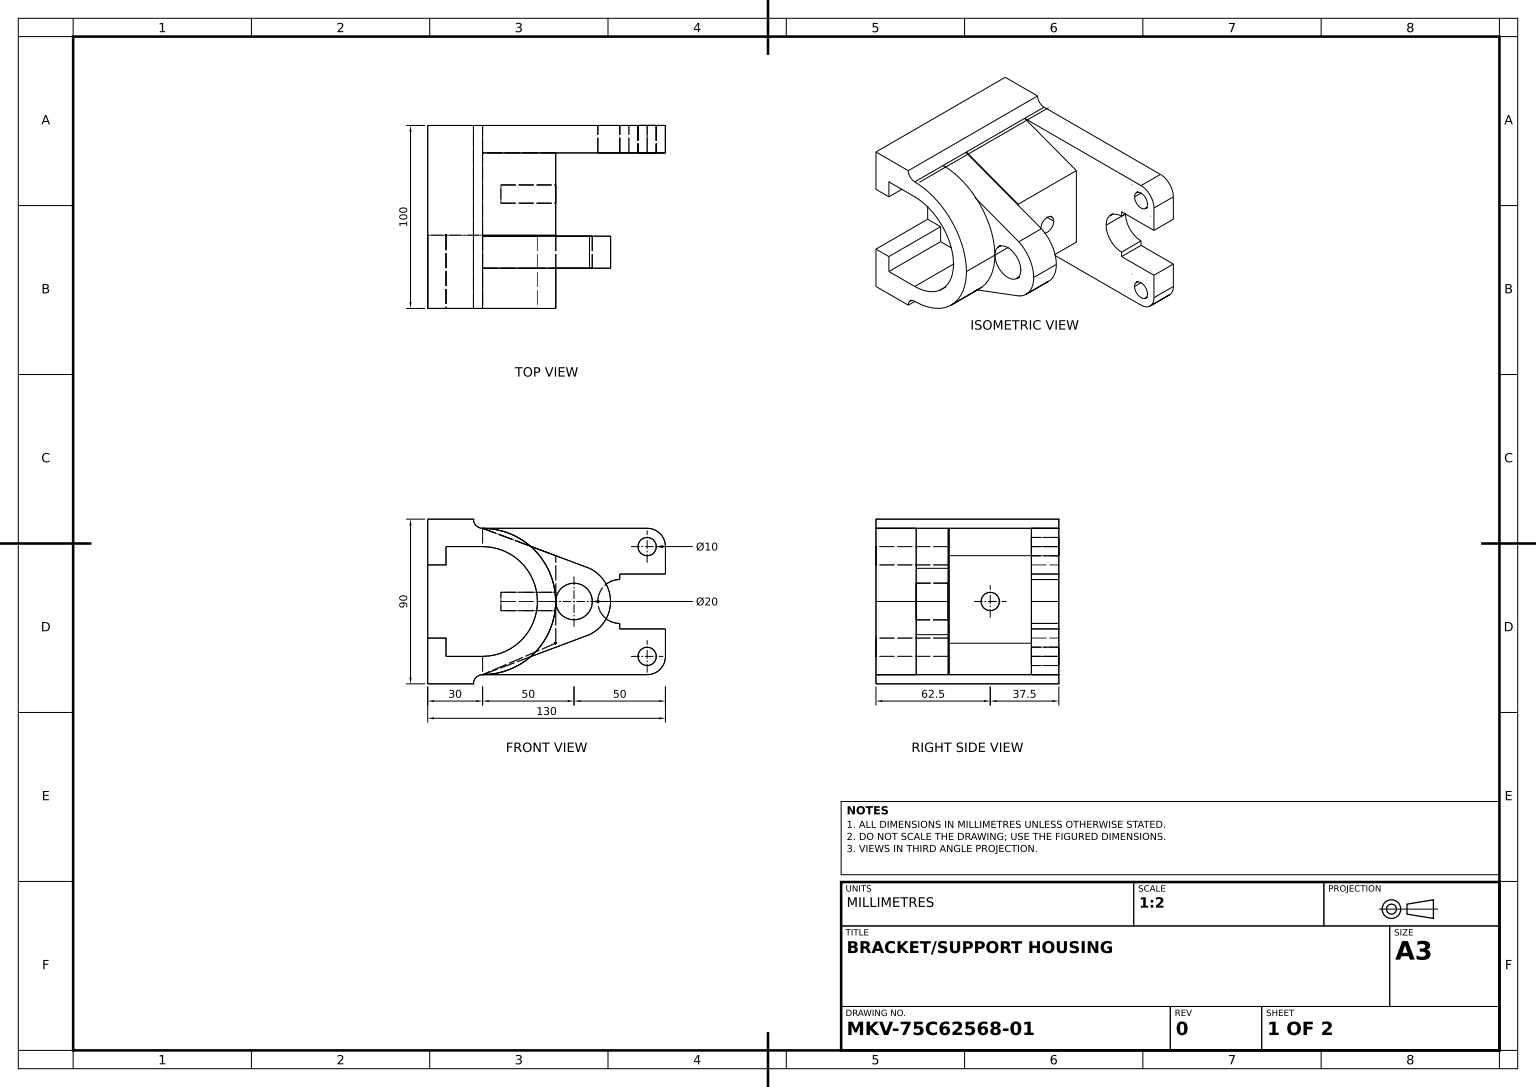
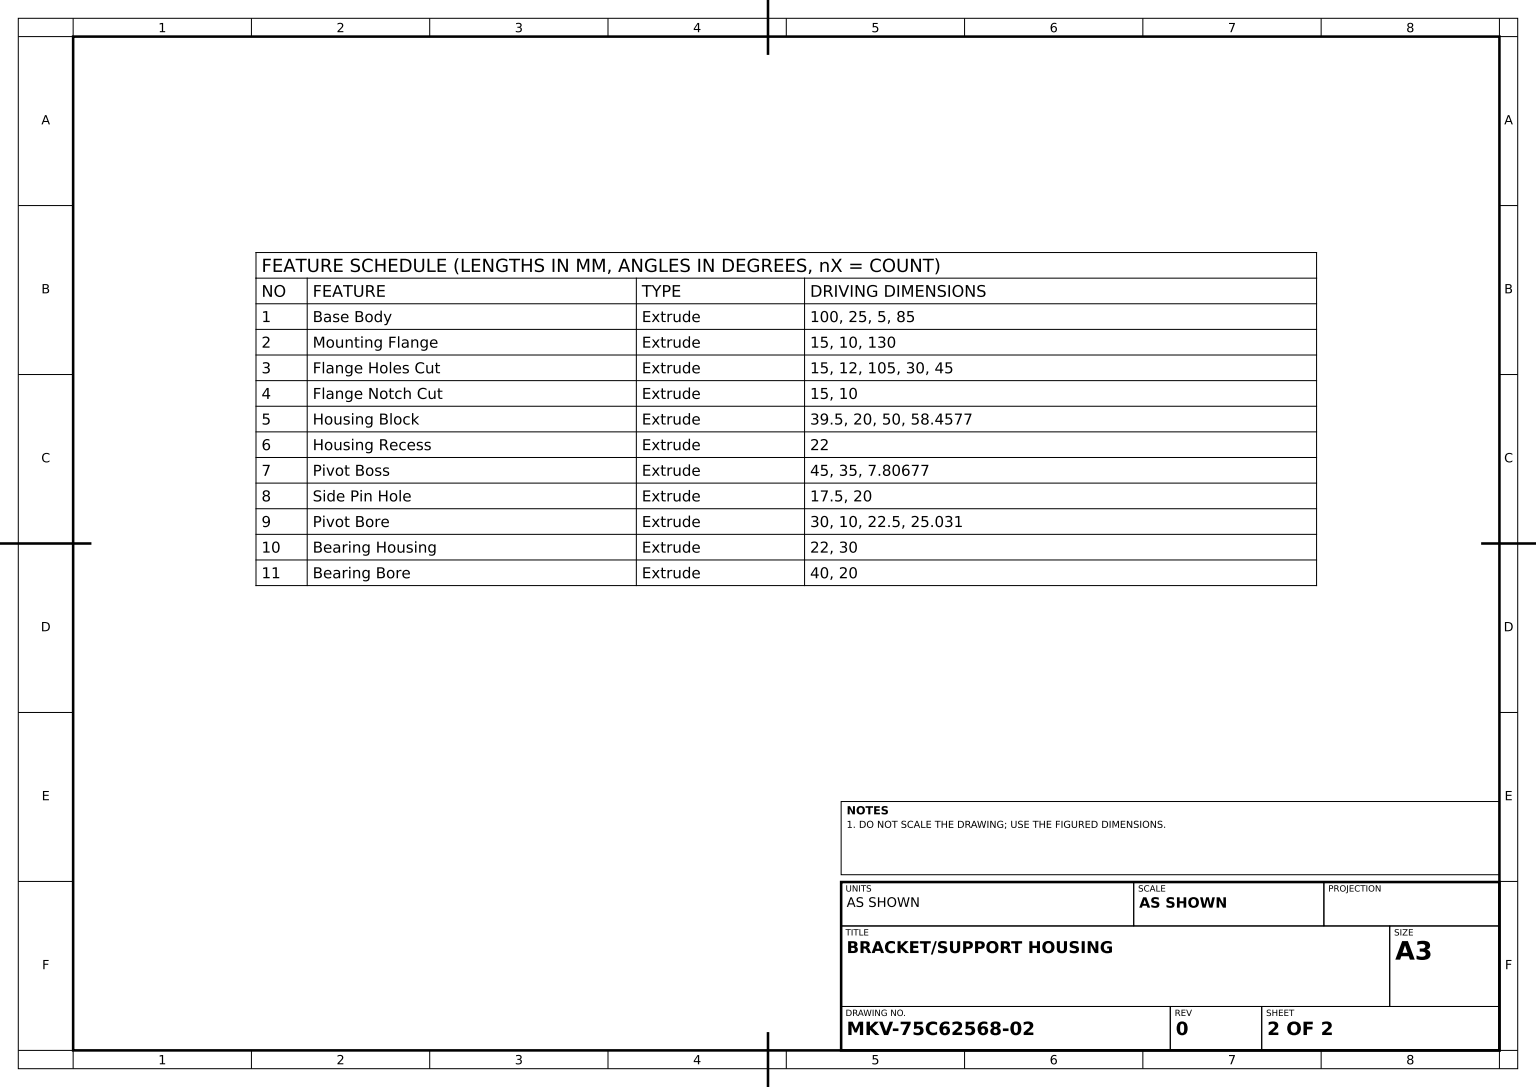
ISO-10303-21;
HEADER;
FILE_DESCRIPTION((''),'2;1');
FILE_NAME('','',(''),(''),'','','');
FILE_SCHEMA(('AUTOMOTIVE_DESIGN'));
ENDSEC;
DATA;
#1=APPLICATION_CONTEXT('');
#2=PRODUCT_CONTEXT('',#1,'mechanical');
#3=PRODUCT('','','',(#2));
#4=PRODUCT_DEFINITION_FORMATION('','',#3);
#5=PRODUCT_DEFINITION_CONTEXT('',#1,'design');
#6=PRODUCT_DEFINITION('','',#4,#5);
#7=PRODUCT_DEFINITION_SHAPE('','',#6);
#8=(LENGTH_UNIT()NAMED_UNIT(*)SI_UNIT(.MILLI.,.METRE.));
#9=(NAMED_UNIT(*)PLANE_ANGLE_UNIT()SI_UNIT($,.RADIAN.));
#10=(NAMED_UNIT(*)SI_UNIT($,.STERADIAN.)SOLID_ANGLE_UNIT());
#11=UNCERTAINTY_MEASURE_WITH_UNIT(LENGTH_MEASURE(1.E-05),#8,'distance_accuracy_value','');
#12=(GEOMETRIC_REPRESENTATION_CONTEXT(3)GLOBAL_UNCERTAINTY_ASSIGNED_CONTEXT((#11))GLOBAL_UNIT_ASSIGNED_CONTEXT((#8,#9,#10))REPRESENTATION_CONTEXT('',''));
#13=CARTESIAN_POINT('',(10.,15.,100.));
#14=VERTEX_POINT('',#13);
#15=CARTESIAN_POINT('',(30.,15.,100.));
#16=VERTEX_POINT('',#15);
#17=DIRECTION('',(1.,0.,0.));
#18=VECTOR('',#17,1000.);
#19=LINE('',#15,#18);
#20=EDGE_CURVE('',#14,#16,#19,.T.);
#21=ORIENTED_EDGE('',*,*,#20,.T.);
#22=CARTESIAN_POINT('',(30.,15.,60.5));
#23=VERTEX_POINT('',#22);
#24=CARTESIAN_POINT('',(30.,15.,78.));
#25=DIRECTION('',(0.,0.,1.));
#26=VECTOR('',#25,1000.);
#27=LINE('',#24,#26);
#28=EDGE_CURVE('',#23,#16,#27,.T.);
#29=ORIENTED_EDGE('',*,*,#28,.F.);
#30=CARTESIAN_POINT('',(30.,15.,60.));
#31=VERTEX_POINT('',#30);
#32=LINE('',#30,#26);
#33=EDGE_CURVE('',#31,#23,#32,.T.);
#34=ORIENTED_EDGE('',*,*,#33,.F.);
#35=CARTESIAN_POINT('',(10.,15.,60.));
#36=VERTEX_POINT('',#35);
#37=LINE('',#30,#18);
#38=EDGE_CURVE('',#36,#31,#37,.T.);
#39=ORIENTED_EDGE('',*,*,#38,.F.);
#40=LINE('',#35,#26);
#41=EDGE_CURVE('',#36,#14,#40,.T.);
#42=ORIENTED_EDGE('',*,*,#41,.T.);
#43=EDGE_LOOP('',(#21,#29,#34,#39,#42));
#44=FACE_OUTER_BOUND('',#43,.T.);
#45=DIRECTION('',(0.,-1.,0.));
#46=DIRECTION('',(0.,0.,-1.));
#47=AXIS2_PLACEMENT_3D('',#30,#45,#46);
#48=PLANE('',#47);
#49=ADVANCED_FACE('',(#44),#48,.F.);
#50=CARTESIAN_POINT('',(70.,45.,78.));
#51=VERTEX_POINT('',#50);
#52=CARTESIAN_POINT('',(70.,45.,100.));
#53=VERTEX_POINT('',#52);
#54=LINE('',#50,#26);
#55=EDGE_CURVE('',#51,#53,#54,.T.);
#56=ORIENTED_EDGE('',*,*,#55,.F.);
#57=CARTESIAN_POINT('',(56.260379,75.172711,78.));
#58=VERTEX_POINT('',#57);
#59=CARTESIAN_POINT('',(30.,45.,78.));
#60=AXIS2_PLACEMENT_3D('',#59,#25,#17);
#61=CIRCLE('',#60,40.);
#62=EDGE_CURVE('',#51,#58,#61,.T.);
#63=ORIENTED_EDGE('',*,*,#62,.T.);
#64=CARTESIAN_POINT('',(30.,85.,78.));
#65=VERTEX_POINT('',#64);
#66=EDGE_CURVE('',#58,#65,#61,.T.);
#67=ORIENTED_EDGE('',*,*,#66,.T.);
#68=CARTESIAN_POINT('',(30.,85.,100.));
#69=VERTEX_POINT('',#68);
#70=VECTOR('',#46,1000.);
#71=LINE('',#68,#70);
#72=EDGE_CURVE('',#69,#65,#71,.T.);
#73=ORIENTED_EDGE('',*,*,#72,.F.);
#74=CARTESIAN_POINT('',(30.,45.,100.));
#75=AXIS2_PLACEMENT_3D('',#74,#25,#17);
#76=CIRCLE('',#75,40.);
#77=EDGE_CURVE('',#53,#69,#76,.T.);
#78=ORIENTED_EDGE('',*,*,#77,.F.);
#79=EDGE_LOOP('',(#56,#63,#67,#73,#78));
#80=FACE_OUTER_BOUND('',#79,.T.);
#81=CYLINDRICAL_SURFACE('',#60,40.);
#82=ADVANCED_FACE('',(#80),#81,.T.);
#83=CARTESIAN_POINT('',(0.,90.,100.));
#84=VERTEX_POINT('',#83);
#85=CARTESIAN_POINT('',(0.,90.,0.));
#86=VERTEX_POINT('',#85);
#87=LINE('',#83,#70);
#88=EDGE_CURVE('',#84,#86,#87,.T.);
#89=ORIENTED_EDGE('',*,*,#88,.F.);
#90=CARTESIAN_POINT('',(25.,90.,100.));
#91=VERTEX_POINT('',#90);
#92=DIRECTION('',(-1.,0.,0.));
#93=VECTOR('',#92,1000.);
#94=LINE('',#83,#93);
#95=EDGE_CURVE('',#91,#84,#94,.T.);
#96=ORIENTED_EDGE('',*,*,#95,.F.);
#97=CARTESIAN_POINT('',(25.,90.,0.));
#98=VERTEX_POINT('',#97);
#99=LINE('',#90,#70);
#100=EDGE_CURVE('',#91,#98,#99,.T.);
#101=ORIENTED_EDGE('',*,*,#100,.T.);
#102=LINE('',#85,#93);
#103=EDGE_CURVE('',#98,#86,#102,.T.);
#104=ORIENTED_EDGE('',*,*,#103,.T.);
#105=EDGE_LOOP('',(#89,#96,#101,#104));
#106=FACE_OUTER_BOUND('',#105,.T.);
#107=AXIS2_PLACEMENT_3D('',#83,#45,#46);
#108=PLANE('',#107);
#109=ADVANCED_FACE('',(#106),#108,.F.);
#110=CARTESIAN_POINT('',(93.,45.,0.));
#111=VERTEX_POINT('',#110);
#112=CARTESIAN_POINT('',(105.,57.,0.));
#113=VERTEX_POINT('',#112);
#114=CARTESIAN_POINT('',(105.,45.,0.));
#115=AXIS2_PLACEMENT_3D('',#114,#46,#92);
#116=CIRCLE('',#115,12.);
#117=EDGE_CURVE('',#111,#113,#116,.T.);
#118=ORIENTED_EDGE('',*,*,#117,.T.);
#119=CARTESIAN_POINT('',(105.,57.,15.));
#120=VERTEX_POINT('',#119);
#121=LINE('',#119,#70);
#122=EDGE_CURVE('',#120,#113,#121,.T.);
#123=ORIENTED_EDGE('',*,*,#122,.F.);
#124=CARTESIAN_POINT('',(93.,45.,15.));
#125=VERTEX_POINT('',#124);
#126=CARTESIAN_POINT('',(105.,45.,15.));
#127=AXIS2_PLACEMENT_3D('',#126,#46,#92);
#128=CIRCLE('',#127,12.);
#129=EDGE_CURVE('',#125,#120,#128,.T.);
#130=ORIENTED_EDGE('',*,*,#129,.F.);
#131=LINE('',#124,#70);
#132=EDGE_CURVE('',#125,#111,#131,.T.);
#133=ORIENTED_EDGE('',*,*,#132,.T.);
#134=EDGE_LOOP('',(#118,#123,#130,#133));
#135=FACE_OUTER_BOUND('',#134,.T.);
#136=CYLINDRICAL_SURFACE('',#127,12.);
#137=ADVANCED_FACE('',(#135),#136,.F.);
#138=CARTESIAN_POINT('',(30.,85.,0.));
#139=VERTEX_POINT('',#138);
#140=CARTESIAN_POINT('',(120.,85.,0.));
#141=VERTEX_POINT('',#140);
#142=LINE('',#140,#18);
#143=EDGE_CURVE('',#139,#141,#142,.T.);
#144=ORIENTED_EDGE('',*,*,#143,.F.);
#145=CARTESIAN_POINT('',(30.,85.,15.));
#146=VERTEX_POINT('',#145);
#147=LINE('',#145,#70);
#148=EDGE_CURVE('',#146,#139,#147,.T.);
#149=ORIENTED_EDGE('',*,*,#148,.F.);
#150=CARTESIAN_POINT('',(120.,85.,15.));
#151=VERTEX_POINT('',#150);
#152=LINE('',#150,#18);
#153=EDGE_CURVE('',#146,#151,#152,.T.);
#154=ORIENTED_EDGE('',*,*,#153,.T.);
#155=LINE('',#150,#70);
#156=EDGE_CURVE('',#151,#141,#155,.T.);
#157=ORIENTED_EDGE('',*,*,#156,.T.);
#158=EDGE_LOOP('',(#144,#149,#154,#157));
#159=FACE_OUTER_BOUND('',#158,.T.);
#160=DIRECTION('',(0.,1.,0.));
#161=AXIS2_PLACEMENT_3D('',#150,#160,#25);
#162=PLANE('',#161);
#163=ADVANCED_FACE('',(#159),#162,.T.);
#164=CARTESIAN_POINT('',(0.,65.,100.));
#165=VERTEX_POINT('',#164);
#166=CARTESIAN_POINT('',(0.,0.,100.));
#167=VECTOR('',#45,1000.);
#168=LINE('',#166,#167);
#169=EDGE_CURVE('',#84,#165,#168,.T.);
#170=ORIENTED_EDGE('',*,*,#169,.F.);
#171=ORIENTED_EDGE('',*,*,#88,.T.);
#172=CARTESIAN_POINT('',(0.,0.,0.));
#173=VERTEX_POINT('',#172);
#174=LINE('',#172,#167);
#175=EDGE_CURVE('',#86,#173,#174,.T.);
#176=ORIENTED_EDGE('',*,*,#175,.T.);
#177=VERTEX_POINT('',#166);
#178=LINE('',#166,#70);
#179=EDGE_CURVE('',#177,#173,#178,.T.);
#180=ORIENTED_EDGE('',*,*,#179,.F.);
#181=CARTESIAN_POINT('',(0.,25.,100.));
#182=VERTEX_POINT('',#181);
#183=EDGE_CURVE('',#182,#177,#168,.T.);
#184=ORIENTED_EDGE('',*,*,#183,.F.);
#185=CARTESIAN_POINT('',(0.,25.,60.));
#186=VERTEX_POINT('',#185);
#187=LINE('',#185,#26);
#188=EDGE_CURVE('',#186,#182,#187,.T.);
#189=ORIENTED_EDGE('',*,*,#188,.F.);
#190=CARTESIAN_POINT('',(0.,65.,60.));
#191=VERTEX_POINT('',#190);
#192=LINE('',#185,#167);
#193=EDGE_CURVE('',#191,#186,#192,.T.);
#194=ORIENTED_EDGE('',*,*,#193,.F.);
#195=LINE('',#190,#26);
#196=EDGE_CURVE('',#191,#165,#195,.T.);
#197=ORIENTED_EDGE('',*,*,#196,.T.);
#198=EDGE_LOOP('',(#170,#171,#176,#180,#184,#189,#194,#197));
#199=FACE_OUTER_BOUND('',#198,.T.);
#200=AXIS2_PLACEMENT_3D('',#166,#17,#46);
#201=PLANE('',#200);
#202=ADVANCED_FACE('',(#199),#201,.F.);
#203=CARTESIAN_POINT('',(70.,22.193233,15.));
#204=VERTEX_POINT('',#203);
#205=CARTESIAN_POINT('',(30.,5.,15.));
#206=VERTEX_POINT('',#205);
#207=CARTESIAN_POINT('',(2.864291,-6.663764,15.));
#208=DIRECTION('',(-0.918725582,-0.394896576,0.));
#209=VECTOR('',#208,1000.);
#210=LINE('',#207,#209);
#211=EDGE_CURVE('',#204,#206,#210,.T.);
#212=ORIENTED_EDGE('',*,*,#211,.F.);
#213=CARTESIAN_POINT('',(70.,22.193233,60.));
#214=VERTEX_POINT('',#213);
#215=LINE('',#213,#70);
#216=EDGE_CURVE('',#214,#204,#215,.T.);
#217=ORIENTED_EDGE('',*,*,#216,.F.);
#218=CARTESIAN_POINT('',(30.,5.,60.));
#219=VERTEX_POINT('',#218);
#220=CARTESIAN_POINT('',(2.864291,-6.663764,60.));
#221=LINE('',#220,#209);
#222=EDGE_CURVE('',#214,#219,#221,.T.);
#223=ORIENTED_EDGE('',*,*,#222,.T.);
#224=LINE('',#218,#70);
#225=EDGE_CURVE('',#219,#206,#224,.T.);
#226=ORIENTED_EDGE('',*,*,#225,.T.);
#227=EDGE_LOOP('',(#212,#217,#223,#226));
#228=FACE_OUTER_BOUND('',#227,.T.);
#229=DIRECTION('',(0.394896576,-0.918725582,0.));
#230=DIRECTION('',(0.918725582,0.394896576,0.));
#231=AXIS2_PLACEMENT_3D('',#220,#229,#230);
#232=PLANE('',#231);
#233=ADVANCED_FACE('',(#228),#232,.T.);
#234=CARTESIAN_POINT('',(105.,60.,0.));
#235=VERTEX_POINT('',#234);
#236=CARTESIAN_POINT('',(130.,60.,0.));
#237=VERTEX_POINT('',#236);
#238=LINE('',#234,#18);
#239=EDGE_CURVE('',#235,#237,#238,.T.);
#240=ORIENTED_EDGE('',*,*,#239,.T.);
#241=CARTESIAN_POINT('',(130.,60.,15.));
#242=VERTEX_POINT('',#241);
#243=LINE('',#241,#70);
#244=EDGE_CURVE('',#242,#237,#243,.T.);
#245=ORIENTED_EDGE('',*,*,#244,.F.);
#246=CARTESIAN_POINT('',(105.,60.,15.));
#247=VERTEX_POINT('',#246);
#248=LINE('',#246,#18);
#249=EDGE_CURVE('',#247,#242,#248,.T.);
#250=ORIENTED_EDGE('',*,*,#249,.F.);
#251=LINE('',#246,#70);
#252=EDGE_CURVE('',#247,#235,#251,.T.);
#253=ORIENTED_EDGE('',*,*,#252,.T.);
#254=EDGE_LOOP('',(#240,#245,#250,#253));
#255=FACE_OUTER_BOUND('',#254,.T.);
#256=AXIS2_PLACEMENT_3D('',#246,#160,#25);
#257=PLANE('',#256);
#258=ADVANCED_FACE('',(#255),#257,.F.);
#259=CARTESIAN_POINT('',(25.,0.,100.));
#260=VERTEX_POINT('',#259);
#261=CARTESIAN_POINT('',(25.,0.,0.));
#262=VERTEX_POINT('',#261);
#263=LINE('',#259,#70);
#264=EDGE_CURVE('',#260,#262,#263,.T.);
#265=ORIENTED_EDGE('',*,*,#264,.F.);
#266=LINE('',#259,#18);
#267=EDGE_CURVE('',#177,#260,#266,.T.);
#268=ORIENTED_EDGE('',*,*,#267,.F.);
#269=ORIENTED_EDGE('',*,*,#179,.T.);
#270=LINE('',#261,#18);
#271=EDGE_CURVE('',#173,#262,#270,.T.);
#272=ORIENTED_EDGE('',*,*,#271,.T.);
#273=EDGE_LOOP('',(#265,#268,#269,#272));
#274=FACE_OUTER_BOUND('',#273,.T.);
#275=AXIS2_PLACEMENT_3D('',#259,#160,#25);
#276=PLANE('',#275);
#277=ADVANCED_FACE('',(#274),#276,.F.);
#278=CARTESIAN_POINT('',(10.,65.,60.));
#279=VERTEX_POINT('',#278);
#280=LINE('',#278,#93);
#281=EDGE_CURVE('',#279,#191,#280,.T.);
#282=ORIENTED_EDGE('',*,*,#281,.F.);
#283=CARTESIAN_POINT('',(10.,65.,100.));
#284=VERTEX_POINT('',#283);
#285=LINE('',#278,#26);
#286=EDGE_CURVE('',#279,#284,#285,.T.);
#287=ORIENTED_EDGE('',*,*,#286,.T.);
#288=LINE('',#283,#93);
#289=EDGE_CURVE('',#284,#165,#288,.T.);
#290=ORIENTED_EDGE('',*,*,#289,.T.);
#291=ORIENTED_EDGE('',*,*,#196,.F.);
#292=EDGE_LOOP('',(#282,#287,#290,#291));
#293=FACE_OUTER_BOUND('',#292,.T.);
#294=AXIS2_PLACEMENT_3D('',#278,#160,#25);
#295=PLANE('',#294);
#296=ADVANCED_FACE('',(#293),#295,.F.);
#297=CARTESIAN_POINT('',(125.,15.,0.));
#298=VERTEX_POINT('',#297);
#299=CARTESIAN_POINT('',(115.,15.,0.));
#300=VERTEX_POINT('',#299);
#301=CARTESIAN_POINT('',(120.,15.,0.));
#302=AXIS2_PLACEMENT_3D('',#301,#25,#17);
#303=CIRCLE('',#302,5.);
#304=EDGE_CURVE('',#298,#300,#303,.T.);
#305=ORIENTED_EDGE('',*,*,#304,.T.);
#306=EDGE_CURVE('',#300,#298,#303,.T.);
#307=ORIENTED_EDGE('',*,*,#306,.T.);
#308=EDGE_LOOP('',(#305,#307));
#309=FACE_BOUND('',#308,.T.);
#310=CARTESIAN_POINT('',(125.,75.,0.));
#311=VERTEX_POINT('',#310);
#312=CARTESIAN_POINT('',(115.,75.,0.));
#313=VERTEX_POINT('',#312);
#314=CARTESIAN_POINT('',(120.,75.,0.));
#315=AXIS2_PLACEMENT_3D('',#314,#25,#17);
#316=CIRCLE('',#315,5.);
#317=EDGE_CURVE('',#311,#313,#316,.T.);
#318=ORIENTED_EDGE('',*,*,#317,.T.);
#319=EDGE_CURVE('',#313,#311,#316,.T.);
#320=ORIENTED_EDGE('',*,*,#319,.T.);
#321=EDGE_LOOP('',(#318,#320));
#322=FACE_BOUND('',#321,.T.);
#323=CARTESIAN_POINT('',(130.,30.,0.));
#324=VERTEX_POINT('',#323);
#325=CARTESIAN_POINT('',(130.,15.,0.));
#326=VERTEX_POINT('',#325);
#327=CARTESIAN_POINT('',(130.,45.,0.));
#328=LINE('',#327,#167);
#329=EDGE_CURVE('',#324,#326,#328,.T.);
#330=ORIENTED_EDGE('',*,*,#329,.T.);
#331=CARTESIAN_POINT('',(120.,5.,0.));
#332=VERTEX_POINT('',#331);
#333=AXIS2_PLACEMENT_3D('',#301,#46,#92);
#334=CIRCLE('',#333,10.);
#335=EDGE_CURVE('',#326,#332,#334,.T.);
#336=ORIENTED_EDGE('',*,*,#335,.T.);
#337=CARTESIAN_POINT('',(30.,5.,0.));
#338=VERTEX_POINT('',#337);
#339=LINE('',#337,#93);
#340=EDGE_CURVE('',#332,#338,#339,.T.);
#341=ORIENTED_EDGE('',*,*,#340,.T.);
#342=CARTESIAN_POINT('',(30.,0.,0.));
#343=AXIS2_PLACEMENT_3D('',#342,#46,#17);
#344=CIRCLE('',#343,5.);
#345=EDGE_CURVE('',#262,#338,#344,.T.);
#346=ORIENTED_EDGE('',*,*,#345,.F.);
#347=ORIENTED_EDGE('',*,*,#271,.F.);
#348=ORIENTED_EDGE('',*,*,#175,.F.);
#349=ORIENTED_EDGE('',*,*,#103,.F.);
#350=CARTESIAN_POINT('',(30.,90.,0.));
#351=AXIS2_PLACEMENT_3D('',#350,#46,#17);
#352=CIRCLE('',#351,5.);
#353=EDGE_CURVE('',#139,#98,#352,.T.);
#354=ORIENTED_EDGE('',*,*,#353,.F.);
#355=ORIENTED_EDGE('',*,*,#143,.T.);
#356=CARTESIAN_POINT('',(130.,75.,0.));
#357=VERTEX_POINT('',#356);
#358=AXIS2_PLACEMENT_3D('',#314,#46,#92);
#359=CIRCLE('',#358,10.);
#360=EDGE_CURVE('',#141,#357,#359,.T.);
#361=ORIENTED_EDGE('',*,*,#360,.T.);
#362=EDGE_CURVE('',#357,#237,#328,.T.);
#363=ORIENTED_EDGE('',*,*,#362,.T.);
#364=ORIENTED_EDGE('',*,*,#239,.F.);
#365=VECTOR('',#160,1000.);
#366=LINE('',#234,#365);
#367=EDGE_CURVE('',#113,#235,#366,.T.);
#368=ORIENTED_EDGE('',*,*,#367,.F.);
#369=ORIENTED_EDGE('',*,*,#117,.F.);
#370=CARTESIAN_POINT('',(105.,33.,0.));
#371=VERTEX_POINT('',#370);
#372=EDGE_CURVE('',#371,#111,#116,.T.);
#373=ORIENTED_EDGE('',*,*,#372,.F.);
#374=CARTESIAN_POINT('',(105.,30.,0.));
#375=VERTEX_POINT('',#374);
#376=LINE('',#370,#365);
#377=EDGE_CURVE('',#375,#371,#376,.T.);
#378=ORIENTED_EDGE('',*,*,#377,.F.);
#379=LINE('',#374,#93);
#380=EDGE_CURVE('',#324,#375,#379,.T.);
#381=ORIENTED_EDGE('',*,*,#380,.F.);
#382=EDGE_LOOP('',(#330,#336,#341,#346,#347,#348,#349,#354,#355,#361,#363,#364,#368,#369,#373,#378,#381));
#383=FACE_OUTER_BOUND('',#382,.T.);
#384=AXIS2_PLACEMENT_3D('',#350,#25,#17);
#385=PLANE('',#384);
#386=ADVANCED_FACE('',(#309,#322,#383),#385,.F.);
#387=CARTESIAN_POINT('',(56.260379,14.827289,78.));
#388=VERTEX_POINT('',#387);
#389=CARTESIAN_POINT('',(88.457667,26.876317,78.));
#390=VERTEX_POINT('',#389);
#391=CARTESIAN_POINT('',(30.,5.,78.));
#392=DIRECTION('',(0.936567609,0.350486966,0.));
#393=VECTOR('',#392,1000.);
#394=LINE('',#391,#393);
#395=EDGE_CURVE('',#388,#390,#394,.T.);
#396=ORIENTED_EDGE('',*,*,#395,.F.);
#397=VERTEX_POINT('',#391);
#398=EDGE_CURVE('',#397,#388,#394,.T.);
#399=ORIENTED_EDGE('',*,*,#398,.F.);
#400=CARTESIAN_POINT('',(30.,5.,60.5));
#401=VERTEX_POINT('',#400);
#402=CARTESIAN_POINT('',(30.,5.,100.));
#403=LINE('',#402,#70);
#404=EDGE_CURVE('',#397,#401,#403,.T.);
#405=ORIENTED_EDGE('',*,*,#404,.T.);
#406=CARTESIAN_POINT('',(88.457667,26.876317,60.5));
#407=VERTEX_POINT('',#406);
#408=LINE('',#400,#393);
#409=EDGE_CURVE('',#401,#407,#408,.T.);
#410=ORIENTED_EDGE('',*,*,#409,.T.);
#411=LINE('',#406,#26);
#412=EDGE_CURVE('',#407,#390,#411,.T.);
#413=ORIENTED_EDGE('',*,*,#412,.T.);
#414=EDGE_LOOP('',(#396,#399,#405,#410,#413));
#415=FACE_OUTER_BOUND('',#414,.T.);
#416=DIRECTION('',(0.350486966,-0.936567609,0.));
#417=AXIS2_PLACEMENT_3D('',#400,#416,#392);
#418=PLANE('',#417);
#419=ADVANCED_FACE('',(#415),#418,.T.);
#420=CARTESIAN_POINT('',(125.,15.,15.));
#421=VERTEX_POINT('',#420);
#422=LINE('',#297,#26);
#423=EDGE_CURVE('',#298,#421,#422,.T.);
#424=ORIENTED_EDGE('',*,*,#423,.T.);
#425=CARTESIAN_POINT('',(115.,15.,15.));
#426=VERTEX_POINT('',#425);
#427=CARTESIAN_POINT('',(120.,15.,15.));
#428=AXIS2_PLACEMENT_3D('',#427,#25,#17);
#429=CIRCLE('',#428,5.);
#430=EDGE_CURVE('',#421,#426,#429,.T.);
#431=ORIENTED_EDGE('',*,*,#430,.T.);
#432=LINE('',#299,#26);
#433=EDGE_CURVE('',#300,#426,#432,.T.);
#434=ORIENTED_EDGE('',*,*,#433,.F.);
#435=ORIENTED_EDGE('',*,*,#304,.F.);
#436=EDGE_LOOP('',(#424,#431,#434,#435));
#437=FACE_OUTER_BOUND('',#436,.T.);
#438=CYLINDRICAL_SURFACE('',#302,5.);
#439=ADVANCED_FACE('',(#437),#438,.F.);
#440=CARTESIAN_POINT('',(30.,75.,60.5));
#441=VERTEX_POINT('',#440);
#442=CARTESIAN_POINT('',(30.,75.,100.));
#443=VERTEX_POINT('',#442);
#444=CARTESIAN_POINT('',(30.,75.,78.));
#445=LINE('',#444,#26);
#446=EDGE_CURVE('',#441,#443,#445,.T.);
#447=ORIENTED_EDGE('',*,*,#446,.F.);
#448=CARTESIAN_POINT('',(60.,45.,60.5));
#449=VERTEX_POINT('',#448);
#450=CARTESIAN_POINT('',(30.,45.,60.5));
#451=AXIS2_PLACEMENT_3D('',#450,#25,#17);
#452=CIRCLE('',#451,30.);
#453=EDGE_CURVE('',#449,#441,#452,.T.);
#454=ORIENTED_EDGE('',*,*,#453,.F.);
#455=CARTESIAN_POINT('',(60.,45.,100.));
#456=VERTEX_POINT('',#455);
#457=CARTESIAN_POINT('',(60.,45.,78.));
#458=LINE('',#457,#26);
#459=EDGE_CURVE('',#449,#456,#458,.T.);
#460=ORIENTED_EDGE('',*,*,#459,.T.);
#461=CIRCLE('',#75,30.);
#462=EDGE_CURVE('',#456,#443,#461,.T.);
#463=ORIENTED_EDGE('',*,*,#462,.T.);
#464=EDGE_LOOP('',(#447,#454,#460,#463));
#465=FACE_OUTER_BOUND('',#464,.T.);
#466=CYLINDRICAL_SURFACE('',#60,30.);
#467=ADVANCED_FACE('',(#465),#466,.F.);
#468=CARTESIAN_POINT('',(105.,30.,15.));
#469=VERTEX_POINT('',#468);
#470=LINE('',#468,#70);
#471=EDGE_CURVE('',#469,#375,#470,.T.);
#472=ORIENTED_EDGE('',*,*,#471,.T.);
#473=ORIENTED_EDGE('',*,*,#377,.T.);
#474=CARTESIAN_POINT('',(105.,33.,15.));
#475=VERTEX_POINT('',#474);
#476=LINE('',#474,#70);
#477=EDGE_CURVE('',#475,#371,#476,.T.);
#478=ORIENTED_EDGE('',*,*,#477,.F.);
#479=LINE('',#474,#365);
#480=EDGE_CURVE('',#469,#475,#479,.T.);
#481=ORIENTED_EDGE('',*,*,#480,.F.);
#482=EDGE_LOOP('',(#472,#473,#478,#481));
#483=FACE_OUTER_BOUND('',#482,.T.);
#484=AXIS2_PLACEMENT_3D('',#474,#92,#25);
#485=PLANE('',#484);
#486=ADVANCED_FACE('',(#483),#485,.F.);
#487=ORIENTED_EDGE('',*,*,#433,.T.);
#488=EDGE_CURVE('',#426,#421,#429,.T.);
#489=ORIENTED_EDGE('',*,*,#488,.T.);
#490=ORIENTED_EDGE('',*,*,#423,.F.);
#491=ORIENTED_EDGE('',*,*,#306,.F.);
#492=EDGE_LOOP('',(#487,#489,#490,#491));
#493=FACE_OUTER_BOUND('',#492,.T.);
#494=ADVANCED_FACE('',(#493),#438,.F.);
#495=ORIENTED_EDGE('',*,*,#395,.T.);
#496=CARTESIAN_POINT('',(100.,45.,78.));
#497=VERTEX_POINT('',#496);
#498=CARTESIAN_POINT('',(80.,45.,78.));
#499=AXIS2_PLACEMENT_3D('',#498,#25,#17);
#500=CIRCLE('',#499,20.);
#501=EDGE_CURVE('',#390,#497,#500,.T.);
#502=ORIENTED_EDGE('',*,*,#501,.T.);
#503=CARTESIAN_POINT('',(88.457667,63.123683,78.));
#504=VERTEX_POINT('',#503);
#505=EDGE_CURVE('',#497,#504,#500,.T.);
#506=ORIENTED_EDGE('',*,*,#505,.T.);
#507=DIRECTION('',(-0.936567609,0.350486966,0.));
#508=VECTOR('',#507,1000.);
#509=LINE('',#503,#508);
#510=EDGE_CURVE('',#504,#58,#509,.T.);
#511=ORIENTED_EDGE('',*,*,#510,.T.);
#512=ORIENTED_EDGE('',*,*,#62,.F.);
#513=CARTESIAN_POINT('',(90.,45.,78.));
#514=VERTEX_POINT('',#513);
#515=CIRCLE('',#499,10.);
#516=EDGE_CURVE('',#514,#51,#515,.T.);
#517=ORIENTED_EDGE('',*,*,#516,.F.);
#518=EDGE_CURVE('',#51,#514,#515,.T.);
#519=ORIENTED_EDGE('',*,*,#518,.F.);
#520=EDGE_CURVE('',#388,#51,#61,.T.);
#521=ORIENTED_EDGE('',*,*,#520,.F.);
#522=EDGE_LOOP('',(#495,#502,#506,#511,#512,#517,#519,#521));
#523=FACE_OUTER_BOUND('',#522,.T.);
#524=PLANE('',#499);
#525=ADVANCED_FACE('',(#523),#524,.T.);
#526=CARTESIAN_POINT('',(125.,75.,15.));
#527=VERTEX_POINT('',#526);
#528=CARTESIAN_POINT('',(115.,75.,15.));
#529=VERTEX_POINT('',#528);
#530=CARTESIAN_POINT('',(120.,75.,15.));
#531=AXIS2_PLACEMENT_3D('',#530,#25,#17);
#532=CIRCLE('',#531,5.);
#533=EDGE_CURVE('',#527,#529,#532,.T.);
#534=ORIENTED_EDGE('',*,*,#533,.T.);
#535=LINE('',#312,#26);
#536=EDGE_CURVE('',#313,#529,#535,.T.);
#537=ORIENTED_EDGE('',*,*,#536,.F.);
#538=ORIENTED_EDGE('',*,*,#317,.F.);
#539=LINE('',#310,#26);
#540=EDGE_CURVE('',#311,#527,#539,.T.);
#541=ORIENTED_EDGE('',*,*,#540,.T.);
#542=EDGE_LOOP('',(#534,#537,#538,#541));
#543=FACE_OUTER_BOUND('',#542,.T.);
#544=CYLINDRICAL_SURFACE('',#315,5.);
#545=ADVANCED_FACE('',(#543),#544,.F.);
#546=CARTESIAN_POINT('',(130.,75.,15.));
#547=VERTEX_POINT('',#546);
#548=AXIS2_PLACEMENT_3D('',#530,#46,#92);
#549=CIRCLE('',#548,10.);
#550=EDGE_CURVE('',#151,#547,#549,.T.);
#551=ORIENTED_EDGE('',*,*,#550,.T.);
#552=LINE('',#546,#70);
#553=EDGE_CURVE('',#547,#357,#552,.T.);
#554=ORIENTED_EDGE('',*,*,#553,.T.);
#555=ORIENTED_EDGE('',*,*,#360,.F.);
#556=ORIENTED_EDGE('',*,*,#156,.F.);
#557=EDGE_LOOP('',(#551,#554,#555,#556));
#558=FACE_OUTER_BOUND('',#557,.T.);
#559=CYLINDRICAL_SURFACE('',#548,10.);
#560=ADVANCED_FACE('',(#558),#559,.T.);
#561=CARTESIAN_POINT('',(30.,85.,60.5));
#562=VERTEX_POINT('',#561);
#563=LINE('',#561,#167);
#564=EDGE_CURVE('',#562,#441,#563,.T.);
#565=ORIENTED_EDGE('',*,*,#564,.T.);
#566=CARTESIAN_POINT('',(30.,75.,60.));
#567=VERTEX_POINT('',#566);
#568=LINE('',#566,#26);
#569=EDGE_CURVE('',#567,#441,#568,.T.);
#570=ORIENTED_EDGE('',*,*,#569,.F.);
#571=CARTESIAN_POINT('',(30.,85.,60.));
#572=VERTEX_POINT('',#571);
#573=CARTESIAN_POINT('',(30.,0.,60.));
#574=LINE('',#573,#167);
#575=EDGE_CURVE('',#572,#567,#574,.T.);
#576=ORIENTED_EDGE('',*,*,#575,.F.);
#577=EDGE_CURVE('',#562,#572,#71,.T.);
#578=ORIENTED_EDGE('',*,*,#577,.F.);
#579=EDGE_LOOP('',(#565,#570,#576,#578));
#580=FACE_OUTER_BOUND('',#579,.T.);
#581=AXIS2_PLACEMENT_3D('',#68,#92,#25);
#582=PLANE('',#581);
#583=ADVANCED_FACE('',(#580),#582,.F.);
#584=CARTESIAN_POINT('',(40.,45.,42.5));
#585=VERTEX_POINT('',#584);
#586=CARTESIAN_POINT('',(40.,45.,32.5));
#587=VERTEX_POINT('',#586);
#588=CARTESIAN_POINT('',(40.,45.,37.5));
#589=AXIS2_PLACEMENT_3D('',#588,#17,#46);
#590=CIRCLE('',#589,5.);
#591=EDGE_CURVE('',#585,#587,#590,.T.);
#592=ORIENTED_EDGE('',*,*,#591,.F.);
#593=CARTESIAN_POINT('',(70.,45.,42.5));
#594=VERTEX_POINT('',#593);
#595=LINE('',#584,#18);
#596=EDGE_CURVE('',#585,#594,#595,.T.);
#597=ORIENTED_EDGE('',*,*,#596,.T.);
#598=CARTESIAN_POINT('',(70.,45.,32.5));
#599=VERTEX_POINT('',#598);
#600=CARTESIAN_POINT('',(70.,45.,37.5));
#601=AXIS2_PLACEMENT_3D('',#600,#17,#46);
#602=CIRCLE('',#601,5.);
#603=EDGE_CURVE('',#594,#599,#602,.T.);
#604=ORIENTED_EDGE('',*,*,#603,.T.);
#605=LINE('',#586,#18);
#606=EDGE_CURVE('',#587,#599,#605,.T.);
#607=ORIENTED_EDGE('',*,*,#606,.F.);
#608=EDGE_LOOP('',(#592,#597,#604,#607));
#609=FACE_OUTER_BOUND('',#608,.T.);
#610=CYLINDRICAL_SURFACE('',#589,5.);
#611=ADVANCED_FACE('',(#609),#610,.F.);
#612=CARTESIAN_POINT('',(70.,70.031002,60.));
#613=VERTEX_POINT('',#612);
#614=CARTESIAN_POINT('',(70.,70.031002,15.));
#615=VERTEX_POINT('',#614);
#616=LINE('',#612,#70);
#617=EDGE_CURVE('',#613,#615,#616,.T.);
#618=ORIENTED_EDGE('',*,*,#617,.T.);
#619=CARTESIAN_POINT('',(31.586886,84.406148,15.));
#620=LINE('',#619,#508);
#621=EDGE_CURVE('',#615,#146,#620,.T.);
#622=ORIENTED_EDGE('',*,*,#621,.T.);
#623=LINE('',#571,#70);
#624=EDGE_CURVE('',#572,#146,#623,.T.);
#625=ORIENTED_EDGE('',*,*,#624,.F.);
#626=CARTESIAN_POINT('',(31.586886,84.406148,60.));
#627=LINE('',#626,#508);
#628=EDGE_CURVE('',#613,#572,#627,.T.);
#629=ORIENTED_EDGE('',*,*,#628,.F.);
#630=EDGE_LOOP('',(#618,#622,#625,#629));
#631=FACE_OUTER_BOUND('',#630,.T.);
#632=DIRECTION('',(-0.350486966,-0.936567609,0.));
#633=DIRECTION('',(0.936567609,-0.350486966,0.));
#634=AXIS2_PLACEMENT_3D('',#626,#632,#633);
#635=PLANE('',#634);
#636=ADVANCED_FACE('',(#631),#635,.F.);
#637=ORIENTED_EDGE('',*,*,#329,.F.);
#638=CARTESIAN_POINT('',(130.,30.,15.));
#639=VERTEX_POINT('',#638);
#640=LINE('',#638,#70);
#641=EDGE_CURVE('',#639,#324,#640,.T.);
#642=ORIENTED_EDGE('',*,*,#641,.F.);
#643=CARTESIAN_POINT('',(130.,15.,15.));
#644=VERTEX_POINT('',#643);
#645=CARTESIAN_POINT('',(130.,45.,15.));
#646=LINE('',#645,#167);
#647=EDGE_CURVE('',#639,#644,#646,.T.);
#648=ORIENTED_EDGE('',*,*,#647,.T.);
#649=LINE('',#643,#70);
#650=EDGE_CURVE('',#644,#326,#649,.T.);
#651=ORIENTED_EDGE('',*,*,#650,.T.);
#652=EDGE_LOOP('',(#637,#642,#648,#651));
#653=FACE_OUTER_BOUND('',#652,.T.);
#654=AXIS2_PLACEMENT_3D('',#645,#17,#46);
#655=PLANE('',#654);
#656=ADVANCED_FACE('',(#653),#655,.T.);
#657=ORIENTED_EDGE('',*,*,#606,.T.);
#658=EDGE_CURVE('',#599,#594,#602,.T.);
#659=ORIENTED_EDGE('',*,*,#658,.T.);
#660=ORIENTED_EDGE('',*,*,#596,.F.);
#661=EDGE_CURVE('',#587,#585,#590,.T.);
#662=ORIENTED_EDGE('',*,*,#661,.F.);
#663=EDGE_LOOP('',(#657,#659,#660,#662));
#664=FACE_OUTER_BOUND('',#663,.T.);
#665=ADVANCED_FACE('',(#664),#610,.F.);
#666=ORIENTED_EDGE('',*,*,#122,.T.);
#667=ORIENTED_EDGE('',*,*,#367,.T.);
#668=ORIENTED_EDGE('',*,*,#252,.F.);
#669=LINE('',#246,#365);
#670=EDGE_CURVE('',#120,#247,#669,.T.);
#671=ORIENTED_EDGE('',*,*,#670,.F.);
#672=EDGE_LOOP('',(#666,#667,#668,#671));
#673=FACE_OUTER_BOUND('',#672,.T.);
#674=AXIS2_PLACEMENT_3D('',#246,#92,#25);
#675=PLANE('',#674);
#676=ADVANCED_FACE('',(#673),#675,.F.);
#677=CARTESIAN_POINT('',(10.,75.,60.));
#678=VERTEX_POINT('',#677);
#679=CARTESIAN_POINT('',(10.,75.,100.));
#680=VERTEX_POINT('',#679);
#681=LINE('',#677,#26);
#682=EDGE_CURVE('',#678,#680,#681,.T.);
#683=ORIENTED_EDGE('',*,*,#682,.F.);
#684=LINE('',#566,#93);
#685=EDGE_CURVE('',#567,#678,#684,.T.);
#686=ORIENTED_EDGE('',*,*,#685,.F.);
#687=ORIENTED_EDGE('',*,*,#569,.T.);
#688=ORIENTED_EDGE('',*,*,#446,.T.);
#689=LINE('',#442,#93);
#690=EDGE_CURVE('',#443,#680,#689,.T.);
#691=ORIENTED_EDGE('',*,*,#690,.T.);
#692=EDGE_LOOP('',(#683,#686,#687,#688,#691));
#693=FACE_OUTER_BOUND('',#692,.T.);
#694=AXIS2_PLACEMENT_3D('',#566,#160,#25);
#695=PLANE('',#694);
#696=ADVANCED_FACE('',(#693),#695,.F.);
#697=EDGE_CURVE('',#23,#449,#452,.T.);
#698=ORIENTED_EDGE('',*,*,#697,.T.);
#699=ORIENTED_EDGE('',*,*,#453,.T.);
#700=ORIENTED_EDGE('',*,*,#564,.F.);
#701=CARTESIAN_POINT('',(88.457667,63.123683,60.5));
#702=VERTEX_POINT('',#701);
#703=LINE('',#561,#508);
#704=EDGE_CURVE('',#702,#562,#703,.T.);
#705=ORIENTED_EDGE('',*,*,#704,.F.);
#706=CARTESIAN_POINT('',(100.,45.,60.5));
#707=VERTEX_POINT('',#706);
#708=CARTESIAN_POINT('',(80.,45.,60.5));
#709=AXIS2_PLACEMENT_3D('',#708,#25,#17);
#710=CIRCLE('',#709,20.);
#711=EDGE_CURVE('',#707,#702,#710,.T.);
#712=ORIENTED_EDGE('',*,*,#711,.F.);
#713=EDGE_CURVE('',#407,#707,#710,.T.);
#714=ORIENTED_EDGE('',*,*,#713,.F.);
#715=ORIENTED_EDGE('',*,*,#409,.F.);
#716=EDGE_CURVE('',#23,#401,#563,.T.);
#717=ORIENTED_EDGE('',*,*,#716,.F.);
#718=EDGE_LOOP('',(#698,#699,#700,#705,#712,#714,#715,#717));
#719=FACE_OUTER_BOUND('',#718,.T.);
#720=CARTESIAN_POINT('',(70.,45.,60.5));
#721=VERTEX_POINT('',#720);
#722=CARTESIAN_POINT('',(90.,45.,60.5));
#723=VERTEX_POINT('',#722);
#724=CIRCLE('',#709,10.);
#725=EDGE_CURVE('',#721,#723,#724,.T.);
#726=ORIENTED_EDGE('',*,*,#725,.T.);
#727=EDGE_CURVE('',#723,#721,#724,.T.);
#728=ORIENTED_EDGE('',*,*,#727,.T.);
#729=EDGE_LOOP('',(#726,#728));
#730=FACE_BOUND('',#729,.T.);
#731=PLANE('',#709);
#732=ADVANCED_FACE('',(#719,#730),#731,.F.);
#733=ORIENTED_EDGE('',*,*,#471,.F.);
#734=LINE('',#468,#93);
#735=EDGE_CURVE('',#639,#469,#734,.T.);
#736=ORIENTED_EDGE('',*,*,#735,.F.);
#737=ORIENTED_EDGE('',*,*,#641,.T.);
#738=ORIENTED_EDGE('',*,*,#380,.T.);
#739=EDGE_LOOP('',(#733,#736,#737,#738));
#740=FACE_OUTER_BOUND('',#739,.T.);
#741=AXIS2_PLACEMENT_3D('',#468,#45,#17);
#742=PLANE('',#741);
#743=ADVANCED_FACE('',(#740),#742,.F.);
#744=ORIENTED_EDGE('',*,*,#682,.T.);
#745=LINE('',#679,#167);
#746=EDGE_CURVE('',#680,#284,#745,.T.);
#747=ORIENTED_EDGE('',*,*,#746,.T.);
#748=ORIENTED_EDGE('',*,*,#286,.F.);
#749=LINE('',#677,#167);
#750=EDGE_CURVE('',#678,#279,#749,.T.);
#751=ORIENTED_EDGE('',*,*,#750,.F.);
#752=EDGE_LOOP('',(#744,#747,#748,#751));
#753=FACE_OUTER_BOUND('',#752,.T.);
#754=AXIS2_PLACEMENT_3D('',#677,#92,#25);
#755=PLANE('',#754);
#756=ADVANCED_FACE('',(#753),#755,.F.);
#757=EDGE_CURVE('',#397,#388,#61,.T.);
#758=ORIENTED_EDGE('',*,*,#757,.F.);
#759=ORIENTED_EDGE('',*,*,#398,.T.);
#760=EDGE_LOOP('',(#758,#759));
#761=FACE_OUTER_BOUND('',#760,.T.);
#762=CARTESIAN_POINT('',(0.,0.,78.));
#763=AXIS2_PLACEMENT_3D('',#762,#25,#17);
#764=PLANE('',#763);
#765=ADVANCED_FACE('',(#761),#764,.F.);
#766=ORIENTED_EDGE('',*,*,#727,.F.);
#767=LINE('',#722,#26);
#768=EDGE_CURVE('',#723,#514,#767,.T.);
#769=ORIENTED_EDGE('',*,*,#768,.T.);
#770=ORIENTED_EDGE('',*,*,#516,.T.);
#771=LINE('',#720,#26);
#772=EDGE_CURVE('',#721,#51,#771,.T.);
#773=ORIENTED_EDGE('',*,*,#772,.F.);
#774=EDGE_LOOP('',(#766,#769,#770,#773));
#775=FACE_OUTER_BOUND('',#774,.T.);
#776=CYLINDRICAL_SURFACE('',#709,10.);
#777=ADVANCED_FACE('',(#775),#776,.F.);
#778=ORIENTED_EDGE('',*,*,#591,.T.);
#779=ORIENTED_EDGE('',*,*,#661,.T.);
#780=EDGE_LOOP('',(#778,#779));
#781=FACE_OUTER_BOUND('',#780,.T.);
#782=PLANE('',#589);
#783=ADVANCED_FACE('',(#781),#782,.T.);
#784=ORIENTED_EDGE('',*,*,#41,.F.);
#785=CARTESIAN_POINT('',(10.,25.,60.));
#786=VERTEX_POINT('',#785);
#787=LINE('',#35,#167);
#788=EDGE_CURVE('',#786,#36,#787,.T.);
#789=ORIENTED_EDGE('',*,*,#788,.F.);
#790=CARTESIAN_POINT('',(10.,25.,100.));
#791=VERTEX_POINT('',#790);
#792=LINE('',#785,#26);
#793=EDGE_CURVE('',#786,#791,#792,.T.);
#794=ORIENTED_EDGE('',*,*,#793,.T.);
#795=LINE('',#13,#167);
#796=EDGE_CURVE('',#791,#14,#795,.T.);
#797=ORIENTED_EDGE('',*,*,#796,.T.);
#798=EDGE_LOOP('',(#784,#789,#794,#797));
#799=FACE_OUTER_BOUND('',#798,.T.);
#800=AXIS2_PLACEMENT_3D('',#35,#92,#25);
#801=PLANE('',#800);
#802=ADVANCED_FACE('',(#799),#801,.F.);
#803=ORIENTED_EDGE('',*,*,#768,.F.);
#804=ORIENTED_EDGE('',*,*,#725,.F.);
#805=ORIENTED_EDGE('',*,*,#772,.T.);
#806=ORIENTED_EDGE('',*,*,#518,.T.);
#807=EDGE_LOOP('',(#803,#804,#805,#806));
#808=FACE_OUTER_BOUND('',#807,.T.);
#809=ADVANCED_FACE('',(#808),#776,.F.);
#810=EDGE_CURVE('',#31,#219,#574,.T.);
#811=ORIENTED_EDGE('',*,*,#810,.F.);
#812=ORIENTED_EDGE('',*,*,#33,.T.);
#813=ORIENTED_EDGE('',*,*,#716,.T.);
#814=EDGE_CURVE('',#401,#219,#403,.T.);
#815=ORIENTED_EDGE('',*,*,#814,.T.);
#816=EDGE_LOOP('',(#811,#812,#813,#815));
#817=FACE_OUTER_BOUND('',#816,.T.);
#818=ADVANCED_FACE('',(#817),#582,.F.);
#819=ORIENTED_EDGE('',*,*,#793,.F.);
#820=LINE('',#785,#18);
#821=EDGE_CURVE('',#186,#786,#820,.T.);
#822=ORIENTED_EDGE('',*,*,#821,.F.);
#823=ORIENTED_EDGE('',*,*,#188,.T.);
#824=LINE('',#790,#18);
#825=EDGE_CURVE('',#182,#791,#824,.T.);
#826=ORIENTED_EDGE('',*,*,#825,.T.);
#827=EDGE_LOOP('',(#819,#822,#823,#826));
#828=FACE_OUTER_BOUND('',#827,.T.);
#829=AXIS2_PLACEMENT_3D('',#785,#45,#17);
#830=PLANE('',#829);
#831=ADVANCED_FACE('',(#828),#830,.F.);
#832=ORIENTED_EDGE('',*,*,#66,.F.);
#833=VECTOR('',#633,1000.);
#834=LINE('',#64,#833);
#835=EDGE_CURVE('',#65,#58,#834,.T.);
#836=ORIENTED_EDGE('',*,*,#835,.F.);
#837=EDGE_LOOP('',(#832,#836));
#838=FACE_OUTER_BOUND('',#837,.T.);
#839=ADVANCED_FACE('',(#838),#764,.F.);
#840=ORIENTED_EDGE('',*,*,#510,.F.);
#841=LINE('',#701,#26);
#842=EDGE_CURVE('',#702,#504,#841,.T.);
#843=ORIENTED_EDGE('',*,*,#842,.F.);
#844=ORIENTED_EDGE('',*,*,#704,.T.);
#845=EDGE_CURVE('',#65,#562,#71,.T.);
#846=ORIENTED_EDGE('',*,*,#845,.F.);
#847=ORIENTED_EDGE('',*,*,#835,.T.);
#848=EDGE_LOOP('',(#840,#843,#844,#846,#847));
#849=FACE_OUTER_BOUND('',#848,.T.);
#850=DIRECTION('',(0.350486966,0.936567609,0.));
#851=AXIS2_PLACEMENT_3D('',#561,#850,#507);
#852=PLANE('',#851);
#853=ADVANCED_FACE('',(#849),#852,.T.);
#854=CARTESIAN_POINT('',(70.,0.,60.));
#855=LINE('',#854,#365);
#856=EDGE_CURVE('',#214,#613,#855,.T.);
#857=ORIENTED_EDGE('',*,*,#856,.T.);
#858=ORIENTED_EDGE('',*,*,#628,.T.);
#859=ORIENTED_EDGE('',*,*,#575,.T.);
#860=ORIENTED_EDGE('',*,*,#685,.T.);
#861=ORIENTED_EDGE('',*,*,#750,.T.);
#862=ORIENTED_EDGE('',*,*,#281,.T.);
#863=ORIENTED_EDGE('',*,*,#193,.T.);
#864=ORIENTED_EDGE('',*,*,#821,.T.);
#865=ORIENTED_EDGE('',*,*,#788,.T.);
#866=ORIENTED_EDGE('',*,*,#38,.T.);
#867=ORIENTED_EDGE('',*,*,#810,.T.);
#868=ORIENTED_EDGE('',*,*,#222,.F.);
#869=EDGE_LOOP('',(#857,#858,#859,#860,#861,#862,#863,#864,#865,#866,#867,#868));
#870=FACE_OUTER_BOUND('',#869,.T.);
#871=CARTESIAN_POINT('',(0.,0.,60.));
#872=AXIS2_PLACEMENT_3D('',#871,#25,#17);
#873=PLANE('',#872);
#874=ADVANCED_FACE('',(#870),#873,.T.);
#875=ORIENTED_EDGE('',*,*,#842,.T.);
#876=ORIENTED_EDGE('',*,*,#505,.F.);
#877=LINE('',#706,#26);
#878=EDGE_CURVE('',#707,#497,#877,.T.);
#879=ORIENTED_EDGE('',*,*,#878,.F.);
#880=ORIENTED_EDGE('',*,*,#711,.T.);
#881=EDGE_LOOP('',(#875,#876,#879,#880));
#882=FACE_OUTER_BOUND('',#881,.T.);
#883=CYLINDRICAL_SURFACE('',#709,20.);
#884=ADVANCED_FACE('',(#882),#883,.T.);
#885=ORIENTED_EDGE('',*,*,#267,.T.);
#886=VERTEX_POINT('',#402);
#887=CARTESIAN_POINT('',(30.,0.,100.));
#888=AXIS2_PLACEMENT_3D('',#887,#46,#17);
#889=CIRCLE('',#888,5.);
#890=EDGE_CURVE('',#260,#886,#889,.T.);
#891=ORIENTED_EDGE('',*,*,#890,.T.);
#892=EDGE_CURVE('',#886,#53,#76,.T.);
#893=ORIENTED_EDGE('',*,*,#892,.T.);
#894=ORIENTED_EDGE('',*,*,#77,.T.);
#895=CARTESIAN_POINT('',(30.,90.,100.));
#896=AXIS2_PLACEMENT_3D('',#895,#46,#17);
#897=CIRCLE('',#896,5.);
#898=EDGE_CURVE('',#69,#91,#897,.T.);
#899=ORIENTED_EDGE('',*,*,#898,.T.);
#900=ORIENTED_EDGE('',*,*,#95,.T.);
#901=ORIENTED_EDGE('',*,*,#169,.T.);
#902=ORIENTED_EDGE('',*,*,#289,.F.);
#903=ORIENTED_EDGE('',*,*,#746,.F.);
#904=ORIENTED_EDGE('',*,*,#690,.F.);
#905=ORIENTED_EDGE('',*,*,#462,.F.);
#906=EDGE_CURVE('',#16,#456,#461,.T.);
#907=ORIENTED_EDGE('',*,*,#906,.F.);
#908=ORIENTED_EDGE('',*,*,#20,.F.);
#909=ORIENTED_EDGE('',*,*,#796,.F.);
#910=ORIENTED_EDGE('',*,*,#825,.F.);
#911=ORIENTED_EDGE('',*,*,#183,.T.);
#912=EDGE_LOOP('',(#885,#891,#893,#894,#899,#900,#901,#902,#903,#904,#905,#907,#908,#909,#910,#911));
#913=FACE_OUTER_BOUND('',#912,.T.);
#914=AXIS2_PLACEMENT_3D('',#895,#25,#17);
#915=PLANE('',#914);
#916=ADVANCED_FACE('',(#913),#915,.T.);
#917=ORIENTED_EDGE('',*,*,#553,.F.);
#918=EDGE_CURVE('',#547,#242,#646,.T.);
#919=ORIENTED_EDGE('',*,*,#918,.T.);
#920=ORIENTED_EDGE('',*,*,#244,.T.);
#921=ORIENTED_EDGE('',*,*,#362,.F.);
#922=EDGE_LOOP('',(#917,#919,#920,#921));
#923=FACE_OUTER_BOUND('',#922,.T.);
#924=ADVANCED_FACE('',(#923),#655,.T.);
#925=CARTESIAN_POINT('',(120.,5.,15.));
#926=VERTEX_POINT('',#925);
#927=AXIS2_PLACEMENT_3D('',#427,#46,#92);
#928=CIRCLE('',#927,10.);
#929=EDGE_CURVE('',#644,#926,#928,.T.);
#930=ORIENTED_EDGE('',*,*,#929,.T.);
#931=LINE('',#925,#70);
#932=EDGE_CURVE('',#926,#332,#931,.T.);
#933=ORIENTED_EDGE('',*,*,#932,.T.);
#934=ORIENTED_EDGE('',*,*,#335,.F.);
#935=ORIENTED_EDGE('',*,*,#650,.F.);
#936=EDGE_LOOP('',(#930,#933,#934,#935));
#937=FACE_OUTER_BOUND('',#936,.T.);
#938=CYLINDRICAL_SURFACE('',#927,10.);
#939=ADVANCED_FACE('',(#937),#938,.T.);
#940=EDGE_CURVE('',#529,#527,#532,.T.);
#941=ORIENTED_EDGE('',*,*,#940,.T.);
#942=ORIENTED_EDGE('',*,*,#540,.F.);
#943=ORIENTED_EDGE('',*,*,#319,.F.);
#944=ORIENTED_EDGE('',*,*,#536,.T.);
#945=EDGE_LOOP('',(#941,#942,#943,#944));
#946=FACE_OUTER_BOUND('',#945,.T.);
#947=ADVANCED_FACE('',(#946),#544,.F.);
#948=ORIENTED_EDGE('',*,*,#603,.F.);
#949=ORIENTED_EDGE('',*,*,#658,.F.);
#950=EDGE_LOOP('',(#948,#949));
#951=FACE_BOUND('',#950,.T.);
#952=CARTESIAN_POINT('',(70.,0.,15.));
#953=LINE('',#952,#365);
#954=EDGE_CURVE('',#204,#615,#953,.T.);
#955=ORIENTED_EDGE('',*,*,#954,.T.);
#956=ORIENTED_EDGE('',*,*,#617,.F.);
#957=ORIENTED_EDGE('',*,*,#856,.F.);
#958=ORIENTED_EDGE('',*,*,#216,.T.);
#959=EDGE_LOOP('',(#955,#956,#957,#958));
#960=FACE_OUTER_BOUND('',#959,.T.);
#961=AXIS2_PLACEMENT_3D('',#854,#92,#25);
#962=PLANE('',#961);
#963=ADVANCED_FACE('',(#951,#960),#962,.F.);
#964=ORIENTED_EDGE('',*,*,#372,.T.);
#965=ORIENTED_EDGE('',*,*,#132,.F.);
#966=EDGE_CURVE('',#475,#125,#128,.T.);
#967=ORIENTED_EDGE('',*,*,#966,.F.);
#968=ORIENTED_EDGE('',*,*,#477,.T.);
#969=EDGE_LOOP('',(#964,#965,#967,#968));
#970=FACE_OUTER_BOUND('',#969,.T.);
#971=ADVANCED_FACE('',(#970),#136,.F.);
#972=ORIENTED_EDGE('',*,*,#713,.T.);
#973=ORIENTED_EDGE('',*,*,#878,.T.);
#974=ORIENTED_EDGE('',*,*,#501,.F.);
#975=ORIENTED_EDGE('',*,*,#412,.F.);
#976=EDGE_LOOP('',(#972,#973,#974,#975));
#977=FACE_OUTER_BOUND('',#976,.T.);
#978=ADVANCED_FACE('',(#977),#883,.T.);
#979=ORIENTED_EDGE('',*,*,#100,.F.);
#980=ORIENTED_EDGE('',*,*,#898,.F.);
#981=ORIENTED_EDGE('',*,*,#72,.T.);
#982=ORIENTED_EDGE('',*,*,#845,.T.);
#983=ORIENTED_EDGE('',*,*,#577,.T.);
#984=ORIENTED_EDGE('',*,*,#624,.T.);
#985=ORIENTED_EDGE('',*,*,#148,.T.);
#986=ORIENTED_EDGE('',*,*,#353,.T.);
#987=EDGE_LOOP('',(#979,#980,#981,#982,#983,#984,#985,#986));
#988=FACE_OUTER_BOUND('',#987,.T.);
#989=AXIS2_PLACEMENT_3D('',#895,#46,#92);
#990=CYLINDRICAL_SURFACE('',#989,5.);
#991=ADVANCED_FACE('',(#988),#990,.F.);
#992=EDGE_CURVE('',#886,#397,#403,.T.);
#993=ORIENTED_EDGE('',*,*,#992,.F.);
#994=ORIENTED_EDGE('',*,*,#890,.F.);
#995=ORIENTED_EDGE('',*,*,#264,.T.);
#996=ORIENTED_EDGE('',*,*,#345,.T.);
#997=LINE('',#205,#70);
#998=EDGE_CURVE('',#206,#338,#997,.T.);
#999=ORIENTED_EDGE('',*,*,#998,.F.);
#1000=ORIENTED_EDGE('',*,*,#225,.F.);
#1001=ORIENTED_EDGE('',*,*,#814,.F.);
#1002=ORIENTED_EDGE('',*,*,#404,.F.);
#1003=EDGE_LOOP('',(#993,#994,#995,#996,#999,#1000,#1001,#1002));
#1004=FACE_OUTER_BOUND('',#1003,.T.);
#1005=AXIS2_PLACEMENT_3D('',#887,#46,#92);
#1006=CYLINDRICAL_SURFACE('',#1005,5.);
#1007=ADVANCED_FACE('',(#1004),#1006,.F.);
#1008=ORIENTED_EDGE('',*,*,#55,.T.);
#1009=ORIENTED_EDGE('',*,*,#892,.F.);
#1010=ORIENTED_EDGE('',*,*,#992,.T.);
#1011=ORIENTED_EDGE('',*,*,#757,.T.);
#1012=ORIENTED_EDGE('',*,*,#520,.T.);
#1013=EDGE_LOOP('',(#1008,#1009,#1010,#1011,#1012));
#1014=FACE_OUTER_BOUND('',#1013,.T.);
#1015=ADVANCED_FACE('',(#1014),#81,.T.);
#1016=ORIENTED_EDGE('',*,*,#697,.F.);
#1017=ORIENTED_EDGE('',*,*,#28,.T.);
#1018=ORIENTED_EDGE('',*,*,#906,.T.);
#1019=ORIENTED_EDGE('',*,*,#459,.F.);
#1020=EDGE_LOOP('',(#1016,#1017,#1018,#1019));
#1021=FACE_OUTER_BOUND('',#1020,.T.);
#1022=ADVANCED_FACE('',(#1021),#466,.F.);
#1023=ORIENTED_EDGE('',*,*,#940,.F.);
#1024=ORIENTED_EDGE('',*,*,#533,.F.);
#1025=EDGE_LOOP('',(#1023,#1024));
#1026=FACE_BOUND('',#1025,.T.);
#1027=ORIENTED_EDGE('',*,*,#430,.F.);
#1028=ORIENTED_EDGE('',*,*,#488,.F.);
#1029=EDGE_LOOP('',(#1027,#1028));
#1030=FACE_BOUND('',#1029,.T.);
#1031=ORIENTED_EDGE('',*,*,#735,.T.);
#1032=ORIENTED_EDGE('',*,*,#480,.T.);
#1033=ORIENTED_EDGE('',*,*,#966,.T.);
#1034=ORIENTED_EDGE('',*,*,#129,.T.);
#1035=ORIENTED_EDGE('',*,*,#670,.T.);
#1036=ORIENTED_EDGE('',*,*,#249,.T.);
#1037=ORIENTED_EDGE('',*,*,#918,.F.);
#1038=ORIENTED_EDGE('',*,*,#550,.F.);
#1039=ORIENTED_EDGE('',*,*,#153,.F.);
#1040=ORIENTED_EDGE('',*,*,#621,.F.);
#1041=ORIENTED_EDGE('',*,*,#954,.F.);
#1042=ORIENTED_EDGE('',*,*,#211,.T.);
#1043=LINE('',#205,#93);
#1044=EDGE_CURVE('',#926,#206,#1043,.T.);
#1045=ORIENTED_EDGE('',*,*,#1044,.F.);
#1046=ORIENTED_EDGE('',*,*,#929,.F.);
#1047=ORIENTED_EDGE('',*,*,#647,.F.);
#1048=EDGE_LOOP('',(#1031,#1032,#1033,#1034,#1035,#1036,#1037,#1038,#1039,#1040,#1041,#1042,#1045,#1046,#1047));
#1049=FACE_OUTER_BOUND('',#1048,.T.);
#1050=PLANE('',#927);
#1051=ADVANCED_FACE('',(#1026,#1030,#1049),#1050,.F.);
#1052=ORIENTED_EDGE('',*,*,#1044,.T.);
#1053=ORIENTED_EDGE('',*,*,#998,.T.);
#1054=ORIENTED_EDGE('',*,*,#340,.F.);
#1055=ORIENTED_EDGE('',*,*,#932,.F.);
#1056=EDGE_LOOP('',(#1052,#1053,#1054,#1055));
#1057=FACE_OUTER_BOUND('',#1056,.T.);
#1058=AXIS2_PLACEMENT_3D('',#205,#45,#17);
#1059=PLANE('',#1058);
#1060=ADVANCED_FACE('',(#1057),#1059,.T.);
#1061=CLOSED_SHELL('',(#49,#82,#109,#137,#163,#202,#233,#258,#277,#296,#386,#419,#439,#467,#486,#494,#525,#545,#560,#583,#611,#636,#656,#665,#676,#696,#732,#743,#756,#765,#777,#783,#802,#809,#818,#831,#839,#853,#874,#884,#916,#924,#939,#947,#963,#971,#978,#991,#1007,#1015,#1022,#1051,#1060));
#1062=MANIFOLD_SOLID_BREP('',#1061);
#1063=ADVANCED_BREP_SHAPE_REPRESENTATION('',(#1062),#12);
#1064=SHAPE_DEFINITION_REPRESENTATION(#7,#1063);
ENDSEC;
END-ISO-10303-21;
